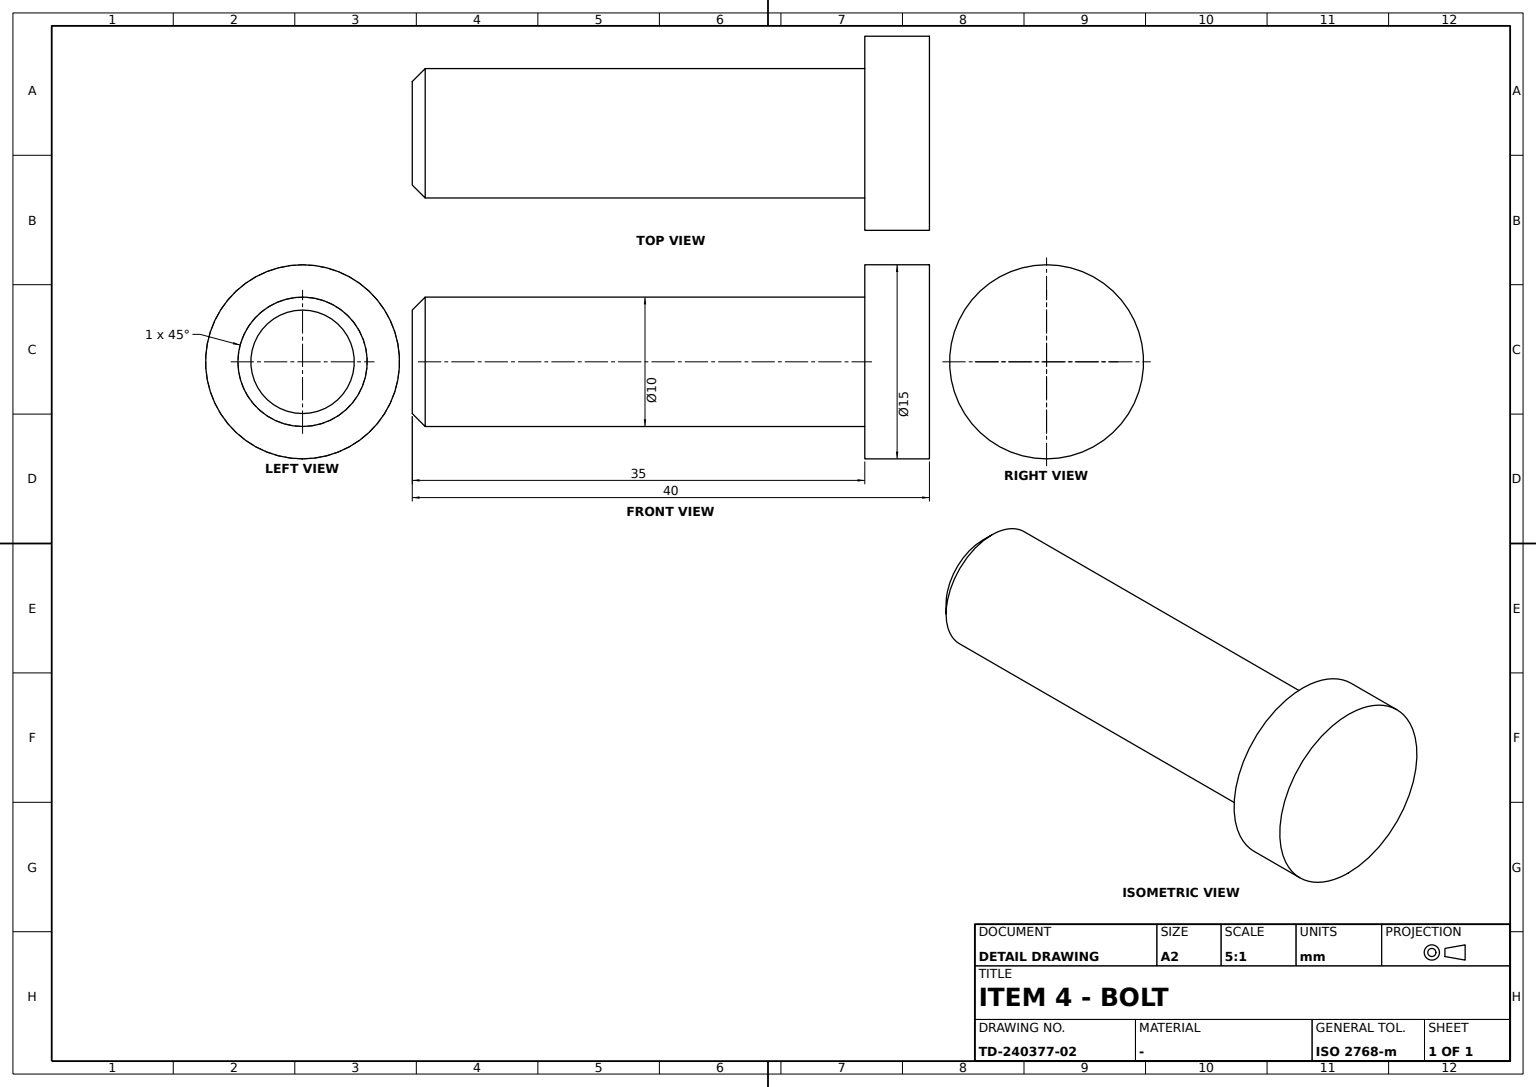
ISO-10303-21;
HEADER;
FILE_DESCRIPTION((''),'2;1');
FILE_NAME('','',(''),(''),'','','');
FILE_SCHEMA(('AUTOMOTIVE_DESIGN'));
ENDSEC;
DATA;
#1=APPLICATION_CONTEXT('');
#2=PRODUCT_CONTEXT('',#1,'mechanical');
#3=PRODUCT('','','',(#2));
#4=PRODUCT_DEFINITION_FORMATION('','',#3);
#5=PRODUCT_DEFINITION_CONTEXT('',#1,'design');
#6=PRODUCT_DEFINITION('','',#4,#5);
#7=PRODUCT_DEFINITION_SHAPE('','',#6);
#8=(LENGTH_UNIT()NAMED_UNIT(*)SI_UNIT(.MILLI.,.METRE.));
#9=(NAMED_UNIT(*)PLANE_ANGLE_UNIT()SI_UNIT($,.RADIAN.));
#10=(NAMED_UNIT(*)SI_UNIT($,.STERADIAN.)SOLID_ANGLE_UNIT());
#11=UNCERTAINTY_MEASURE_WITH_UNIT(LENGTH_MEASURE(0.005),#8,'distance_accuracy_value','');
#12=(GEOMETRIC_REPRESENTATION_CONTEXT(3)GLOBAL_UNCERTAINTY_ASSIGNED_CONTEXT((#11))GLOBAL_UNIT_ASSIGNED_CONTEXT((#8,#9,#10))REPRESENTATION_CONTEXT('',''));
#13=CARTESIAN_POINT('',(0.,0.,-4.));
#14=VERTEX_POINT('',#13);
#15=CARTESIAN_POINT('',(0.,0.,0.));
#16=DIRECTION('',(1.,0.,0.));
#17=DIRECTION('',(0.,0.,-1.));
#18=AXIS2_PLACEMENT_3D('',#15,#16,#17);
#19=CIRCLE('',#18,4.);
#20=EDGE_CURVE('',#14,#14,#19,.T.);
#21=ORIENTED_EDGE('',*,*,#20,.T.);
#22=EDGE_LOOP('',(#21));
#23=FACE_BOUND('',#22,.T.);
#24=CARTESIAN_POINT('',(1.,5.,0.));
#25=VERTEX_POINT('',#24);
#26=CARTESIAN_POINT('',(1.,0.,0.));
#27=DIRECTION('',(0.,1.,0.));
#28=AXIS2_PLACEMENT_3D('',#26,#16,#27);
#29=CIRCLE('',#28,5.);
#30=EDGE_CURVE('',#25,#25,#29,.T.);
#31=ORIENTED_EDGE('',*,*,#30,.F.);
#32=EDGE_LOOP('',(#31));
#33=FACE_BOUND('',#32,.T.);
#34=CARTESIAN_POINT('',(-4.,0.,0.));
#35=DIRECTION('',(0.,-0.95663882,0.291276788));
#36=AXIS2_PLACEMENT_3D('',#34,#16,#35);
#37=CONICAL_SURFACE('',#36,0.,0.785398163);
#38=ADVANCED_FACE('',(#23,#33),#37,.T.);
#39=CARTESIAN_POINT('',(40.,0.,-7.5));
#40=VERTEX_POINT('',#39);
#41=CARTESIAN_POINT('',(40.,0.,0.));
#42=AXIS2_PLACEMENT_3D('',#41,#16,#17);
#43=CIRCLE('',#42,7.5);
#44=EDGE_CURVE('',#40,#40,#43,.T.);
#45=ORIENTED_EDGE('',*,*,#44,.T.);
#46=EDGE_LOOP('',(#45));
#47=FACE_BOUND('',#46,.T.);
#48=AXIS2_PLACEMENT_3D('',#41,#16,#27);
#49=PLANE('',#48);
#50=ADVANCED_FACE('',(#47),#49,.T.);
#51=ORIENTED_EDGE('',*,*,#20,.F.);
#52=EDGE_LOOP('',(#51));
#53=FACE_BOUND('',#52,.T.);
#54=AXIS2_PLACEMENT_3D('',#15,#16,#27);
#55=PLANE('',#54);
#56=ADVANCED_FACE('',(#53),#55,.F.);
#57=CARTESIAN_POINT('',(35.,0.,-7.5));
#58=VERTEX_POINT('',#57);
#59=CARTESIAN_POINT('',(35.,0.,0.));
#60=AXIS2_PLACEMENT_3D('',#59,#16,#17);
#61=CIRCLE('',#60,7.5);
#62=EDGE_CURVE('',#58,#58,#61,.T.);
#63=ORIENTED_EDGE('',*,*,#62,.T.);
#64=EDGE_LOOP('',(#63));
#65=FACE_BOUND('',#64,.T.);
#66=ORIENTED_EDGE('',*,*,#44,.F.);
#67=EDGE_LOOP('',(#66));
#68=FACE_BOUND('',#67,.T.);
#69=CARTESIAN_POINT('',(37.5,0.,0.));
#70=AXIS2_PLACEMENT_3D('',#69,#16,#27);
#71=CYLINDRICAL_SURFACE('',#70,7.5);
#72=ADVANCED_FACE('',(#65,#68),#71,.T.);
#73=CARTESIAN_POINT('',(35.,0.,-5.));
#74=VERTEX_POINT('',#73);
#75=CIRCLE('',#60,5.);
#76=EDGE_CURVE('',#74,#74,#75,.T.);
#77=ORIENTED_EDGE('',*,*,#76,.T.);
#78=EDGE_LOOP('',(#77));
#79=FACE_BOUND('',#78,.T.);
#80=ORIENTED_EDGE('',*,*,#62,.F.);
#81=EDGE_LOOP('',(#80));
#82=FACE_BOUND('',#81,.T.);
#83=AXIS2_PLACEMENT_3D('',#59,#16,#27);
#84=PLANE('',#83);
#85=ADVANCED_FACE('',(#79,#82),#84,.F.);
#86=ORIENTED_EDGE('',*,*,#30,.T.);
#87=EDGE_LOOP('',(#86));
#88=FACE_BOUND('',#87,.T.);
#89=ORIENTED_EDGE('',*,*,#76,.F.);
#90=EDGE_LOOP('',(#89));
#91=FACE_BOUND('',#90,.T.);
#92=CARTESIAN_POINT('',(17.5,0.,0.));
#93=AXIS2_PLACEMENT_3D('',#92,#16,#27);
#94=CYLINDRICAL_SURFACE('',#93,5.);
#95=ADVANCED_FACE('',(#88,#91),#94,.T.);
#96=CLOSED_SHELL('',(#38,#50,#56,#72,#85,#95));
#97=MANIFOLD_SOLID_BREP('',#96);
#98=ADVANCED_BREP_SHAPE_REPRESENTATION('',(#97),#12);
#99=SHAPE_DEFINITION_REPRESENTATION(#7,#98);
ENDSEC;
END-ISO-10303-21;
